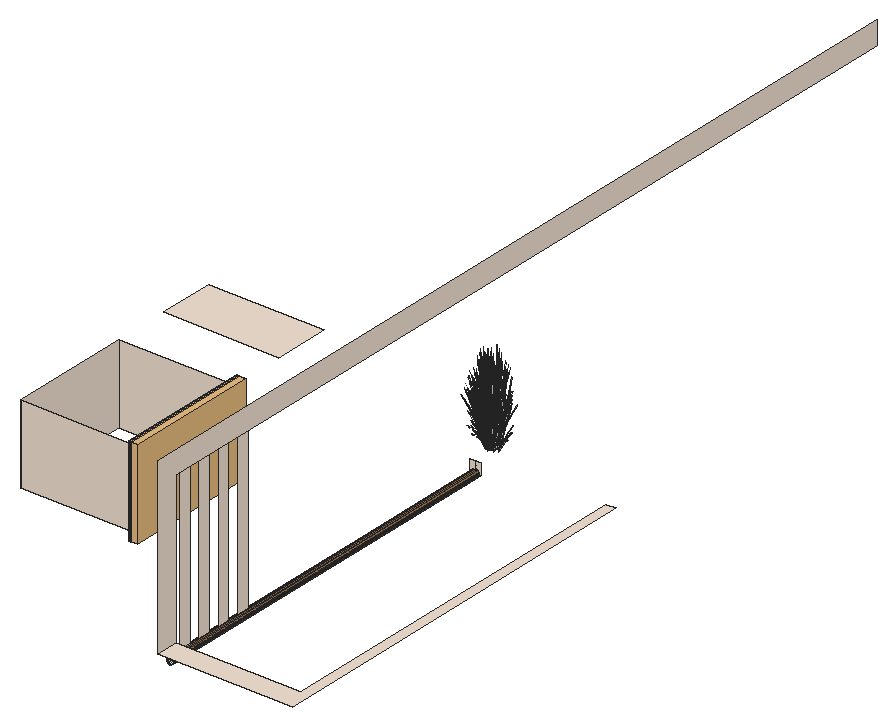
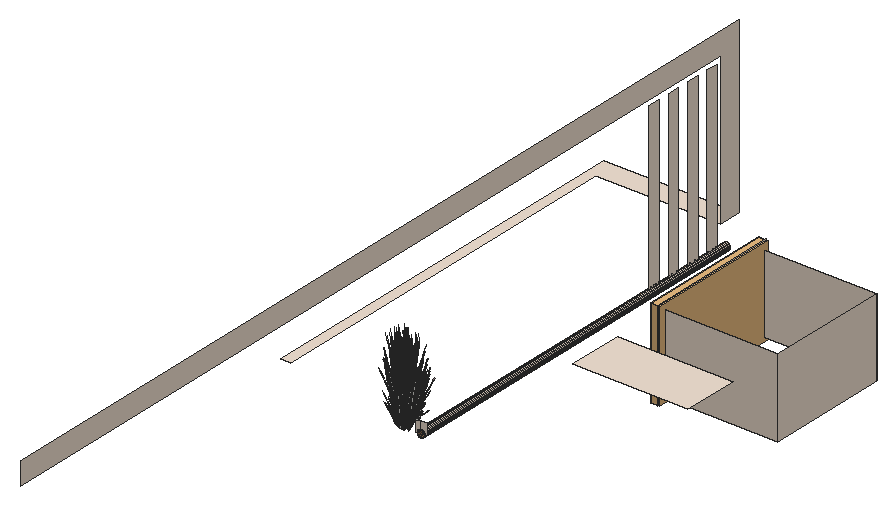
# SketchUp Ruby script. Lengths in inches.
U = 1.inch
M = Sketchup.active_model
def pt(a) = Geom::Point3d.new(a.map { |v| v * U })
def face(e, loops, mat)
  f = e.add_face(loops[0].map { |a| pt(a) })
  loops[1..].each { |l| e.add_face(l.map { |a| pt(a) }).erase! }
  f.material = f.back_material = mat if mat
  f
end
# faces: each face lists its corners as indices into pts; further lists are holes
def faces(e, pts, list, mat = nil) = list.each { |f| face(e, (f[0].is_a?(Array) ? f : [f]).map { |l| l.map { |i| pts[i] } }, mat) }
# xy, xz, yz: faces in a plane at the given z, y or x. An outline is a flat list of corners, or four numbers for a rectangle; further outlines are holes
def ring(l) = l.size == 4 ? [[l[0], l[1]], [l[2], l[1]], [l[2], l[3]], [l[0], l[3]]] : l.each_slice(2).to_a
def flat(e, list, mat, &to3) = list.each { |f| face(e, (f[0].is_a?(Array) ? f : [f]).map { |l| ring(l).map { |u, v| to3.(u, v) } }, mat) }
def xy(e, z, list, mat = nil) = flat(e, list, mat) { |x, y| [x, y, z] }
def xz(e, y, list, mat = nil) = flat(e, list, mat) { |x, z| [x, y, z] }
def yz(e, x, list, mat = nil) = flat(e, list, mat) { |y, z| [x, y, z] }
def lines(e, pts, list) = list.each { |a, b| e.add_line(pt(pts[a]), pt(pts[b])) }
# prism: a flat outline (further loops are holes) pulled along v
def prism(e, loops, v, mat = nil)
  f = face(e, loops, mat); d = Geom::Vector3d.new(v.map { |x| x * U })
  f.pushpull(f.normal.samedirection?(d) ? d.length : -d.length)
end
def box(e, o, s, mat = nil) = prism(e, [[o, [o[0] + s[0], o[1], o[2]], [o[0] + s[0], o[1] + s[1], o[2]], [o[0], o[1] + s[1], o[2]]]], [0, 0, s[2]], mat)
def at(x, y, z, deg = 0) = Geom::Transformation.translation(pt([x, y, z])) * Geom::Transformation.rotation(ORIGIN, Z_AXIS, deg.degrees)
def axes(o, x, y, z) = Geom::Transformation.new([*x, 0, *y, 0, *z, 0, *pt(o).to_a, 1])
def part(name) = M.definitions.add(name)
# library, detail: a bought-in or finely detailed component or shape, given as its bounding box
def library(name, o, s) = part(name).tap { |d| box(d.entities, o, s) }
def detail(e, o, s) = box(e.add_group.entities, o, s)
def put(e, d, t, mat = nil) = e.add_instance(d, t).tap { |i| i.material = mat if mat }
def group(e, t, mat = nil) = e.add_group.tap { |g| g.transformation = t; g.material = mat if mat }.entities
root = M.entities
M.materials.add("C01_Vanilla_Cream").color = [244, 228, 212]
M.materials.add("LightPink_Translucent").color = [144, 107, 117]
M.materials["LightPink_Translucent"].alpha = 0.75
M.materials.add("Wood_Floor_01_1K").color = [146, 111, 76]
c1 = library("Double casement window",[0,0,0],[5.02,56.42,60])
c2 = part("blade")
p = [[2.15,0.21,22],[0,0.17,0],[0.09,0.45,0],[2.18,0.31,22],[2.29,0.31,22],[0.38,0.45,0],
  [2.48,0.24,33],[2.49,0.24,33],[2.48,0.22,33]]
faces(c2.entities,p,[[0,1,2,3],[4,5,2,3],[6,3,4,7],[8,0,3,6]])
c3 = part("seeds")
p = [[0.3,-0.1,1.38],[-0.01,-0.03,1.59],[-0.01,-0.03,0.03],[0.14,-0.07,-0.07],[0.29,-0.03,3],[0.15,0.01,3.11]]
faces(c3.entities,p,[[0,1,2,3],[1,0,4,5]],"LightPink_Translucent")
c4 = part("blade with seeds")
put(c4.entities,c2,at(0,0,0))
put(c4.entities,c3,axes([2.4,0.25,30.99],[1.5799,-0.05474,1.17369],[-0.12525,1.92788,0.29478],[-0.07173,-0.02425,1.56792]))
xy(root,51.56,[[360,0,432,0,432,216,426.72,216,426.72,12,360,12]],"C01_Vanilla_Cream")
xy(root,93,[[226.53,171,288,201]],"C01_Vanilla_Cream")
xz(root,75,[[226.53,51,288,93]],"C01_Vanilla_Cream")
xz(root,141,[[226.53,51,288,93]],"C01_Vanilla_Cream")
xz(root,216,[[354,42,355,42,355.07,42.52,355.27,43,355.59,43.41,356,43.73,356.48,43.93,357,44,357,48,354,48],[359,42,360,42,360,48,357,48,357,44,357.52,43.93,358,43.73,358.41,43.41,358.73,43,358.93,42.52]],"C01_Vanilla_Cream")
yz(root,226.53,[[75,51,141,93]],"C01_Vanilla_Cream")
yz(root,288,[[[72,48,144,96],[109.5,51,141,93],[75,51,106.5,93]]],"C01_Vanilla_Cream")
yz(root,357,[[18.46,40,24.91,44],[31.37,40,37.83,44],[44.28,40,50.74,44],[57.2,40,63.65,44],[18.46,44,24.91,132],
  [31.37,44,37.83,132],[44.28,44,50.74,132],[57.2,44,63.65,132]],"C01_Vanilla_Cream")
yz(root,360,[[0,51.56,12,51.56,12,132,480,132,480,144,0,144]],"C01_Vanilla_Cream")
p = [[356.48,216,40.07],[357,216,40],[357,63.65,40],[357,57.2,40],[357,50.74,40],[357,44.28,40],
  [357,37.83,40],[357,31.37,40],[357,24.91,40],[357,18.46,40],[357,12,40],[356.48,12,40.07],
  [357.52,216,40.07],[357.52,12,40.07],[356,216,40.27],[356,12,40.27],[358,216,40.27],[358,12,40.27],
  [355.59,216,40.59],[355.59,12,40.59],[358.41,216,40.59],[358.41,12,40.59],[355.27,216,41],[355.27,12,41],
  [358.73,216,41],[358.73,12,41],[355.07,216,41.48],[355.07,12,41.48],[358.93,216,41.48],[358.93,12,41.48],
  [355,216,42],[355,12,42],[359,216,42],[359,12,42],[355.07,216,42.52],[355.07,12,42.52],
  [358.93,216,42.52],[358.93,12,42.52],[355.27,216,43],[355.27,12,43],[358.73,216,43],[358.73,12,43],
  [355.59,216,43.41],[355.59,12,43.41],[358.41,216,43.41],[358.41,12,43.41],[356,216,43.73],[356,12,43.73],
  [358,216,43.73],[358,12,43.73],[356.48,216,43.93],[356.48,12,43.93],[357.52,216,43.93],[357.52,12,43.93],
  [357,216,44],[357,12,44],[357,18.46,44],[357,24.91,44],[357,31.37,44],[357,37.83,44],
  [357,44.28,44],[357,50.74,44],[357,57.2,44],[357,63.65,44]]
faces(root,p,[[0,1,2,3,4,5,6,7,8,9,10,11],[14,0,11,15],[18,14,15,19],[22,18,19,23],[26,22,23,27],[30,26,27,31],[34,30,31,35],[38,34,35,39],
  [42,38,39,43],[46,42,43,47],[50,46,47,51],[54,50,51,55,56,57,58,59,60,61,62,63]],"C01_Vanilla_Cream")
faces(root,p,[[1,12,13,10,9,8,7,6,5,4,3,2],[12,16,17,13],[16,20,21,17],[20,24,25,21],[24,28,29,25],[28,32,33,29],[32,36,37,33],[36,40,41,37],
  [40,44,45,41],[44,48,49,45],[48,52,53,49],[52,54,63,62,61,60,59,58,57,56,55,53]],"Wood_Floor_01_1K")
put(root,c1,axes([286.7,72.24,48.3],[1,0,0],[0,1.27666,0],[0,0,0.79394]))
put(root,c4,axes([356.25,225,50.91],[0.12726,0.15818,1.28532],[-0.58807,0.13317,0.10393],[-0.13291,-0.24832,0.54946]))
put(root,c4,axes([357.22,223.95,51.54],[-0.08515,-0.06907,1.31208],[-0.56828,0.04379,-0.2075],[-0.0907,-0.16522,0.10523]))
put(root,c4,axes([358.54,224.77,49.94],[-0.15825,0.09972,1.07251],[-0.47395,-0.17454,-0.23066],[0.08785,-0.21706,0.45856]))
put(root,c4,axes([357.82,225.12,51.74],[-0.26572,-0.40059,-0.53284],[0.54698,-0.22325,0.0643],[-0.06214,-0.19355,0.75375]))
put(root,c4,axes([356.09,224.58,49.94],[-0.03371,0.16116,1.07251],[-0.49286,0.13491,-0.23066],[-0.11521,-0.20831,0.45856]))
put(root,c4,axes([357.36,224.23,49.12],[-0.09338,0.01775,1.32257],[-0.51641,-0.1998,-0.20205],[0.00867,-0.16666,0.22528]))
put(root,c4,axes([358.92,225.51,51.74],[0.01449,-0.45571,-0.53284],[0.61002,0.03061,0.0643],[0.06438,-0.19306,0.75375]))
put(root,c4,axes([359.77,224.8,51.54],[-0.00537,-0.09805,1.31208],[-0.45391,-0.28338,-0.2075],[0.07018,-0.17178,0.10523]))
put(root,c4,axes([357.87,224.78,51.39],[0.16784,-0.37886,-0.2656],[0.48968,0.1105,0.3429],[-0.0449,-0.15254,0.65611]))
put(root,c4,axes([358.24,225.28,50.91],[-0.10366,0.16934,1.28532],[-0.43488,-0.35044,0.10393],[0.19618,-0.21841,0.54946]))
put(root,c4,axes([359.65,224.44,51.53],[-0.05654,0.03763,1.33037],[-0.55396,-0.12696,-0.12571],[-0.02005,-0.16422,0.23543]))
put(root,c4,axes([357.62,225.04,51.51],[-0.54728,-0.1235,-0.38324],[0.18759,-0.42344,-0.29685],[-0.05018,-0.17048,0.7333]))
put(root,c4,axes([357.95,223.98,50.07],[0.07142,0.28728,0.86145],[-0.3962,-0.15911,0.63294],[0.04263,-0.1471,0.18974]))
put(root,c4,axes([358.8,225.36,51.51],[-0.39855,-0.33102,-0.38324],[0.42102,-0.2899,-0.29685],[0.06064,-0.16819,0.7333]))
put(root,c4,axes([356.64,223.72,51.53],[-0.01039,0.05905,1.33037],[-0.51226,0.21431,-0.12571],[-0.15074,-0.10955,0.23543]))
put(root,c4,axes([356.52,224.77,51.82],[0.62019,-0.12663,0.40322],[0.10763,0.49673,0.33247],[-0.14586,-0.1464,0.83437]))
put(root,c4,axes([357.93,224.86,51.55],[0.54859,0.1288,0.36002],[-0.18759,0.42344,0.29685],[-0.03297,-0.16652,0.74497]))
put(root,c4,axes([358.08,225.02,51.78],[-0.54481,0.22937,-0.0912],[-0.26773,-0.4071,-0.50621],[-0.07188,-0.17155,0.76918]))
put(root,c4,axes([359.22,225.53,51.78],[-0.61188,-0.02441,-0.0912],[0.01672,-0.46217,-0.50621],[0.0425,-0.178,0.76918]))
put(root,c4,axes([359.17,225.23,51.39],[0.3767,-0.25939,-0.2656],[0.3566,0.29618,0.3429],[0.05426,-0.15048,0.65611]))
put(root,c4,axes([355.92,224.32,50.07],[0.29042,0.17147,0.86145],[-0.42295,0.10307,0.63294],[-0.0905,-0.13178,0.18974]))
put(root,c4,axes([358.07,224.83,51.55],[0.41024,-0.16744,0.04823],[0.2008,0.30532,0.37966],[-0.03962,-0.13459,0.57892]))
put(root,c4,axes([356.62,225.23,51.74],[-0.47473,-0.23813,-0.53284],[0.33738,-0.41728,0.0643],[-0.172,-0.14218,0.75375]))
put(root,c4,axes([356.45,224.91,51.39],[-0.08599,-0.39682,-0.2656],[0.49155,-0.10478,0.3429],[-0.13203,-0.11372,0.65611]))
put(root,c4,axes([356.67,224.88,51.55],[0.25304,-0.31296,0.04823],[0.36033,0.18221,0.37966],[-0.11649,-0.10034,0.57892]))
put(root,c4,axes([355.6875,224.84,49.12],[-0.05393,0.0649,1.32257],[-0.545,0.13993,-0.20205],[-0.13166,-0.12729,0.22528]))
put(root,c4,axes([356.59,226.62,49.57],[-0.22864,-0.5052,-0.52377],[0.65862,-0.18195,-0.13747],[-0.02527,-0.17107,1.15612]))
put(root,c4,axes([355.4,225.49,50.91],[0.2068,0.08488,1.28532],[-0.42797,0.35609,0.10393],[-0.26673,-0.16064,0.54946]))
put(root,c4,axes([359.64,225.08,49.12],[-0.08333,-0.03881,1.32257],[-0.21404,-0.4336,-0.20205],[0.14439,-0.11767,0.22528]))
put(root,c4,axes([357.92,225.17,51.79],[-0.16784,0.37886,0.2656],[-0.48968,-0.1105,-0.3429],[-0.0449,-0.15254,0.65611]))
put(root,c4,axes([356.4,225.24,51.51],[-0.54938,0.11711,-0.38324],[-0.0961,-0.44351,-0.29685],[-0.14756,-0.1271,0.7333]))
put(root,c4,axes([359.17,225.33,51.55],[0.39645,0.33614,0.36002],[-0.42102,0.2899,0.29685],[0.07313,-0.15771,0.74497]))
put(root,c4,axes([356.78,224.85,52.07],[-0.37157,0.4723,-0.10215],[-0.5381,-0.2721,-0.56695],[-0.18705,-0.13344,0.86148]))
put(root,c4,axes([359.32,225.37,51.55],[0.45752,0.02296,0.04823],[-0.01254,0.34663,0.37966],[0.04787,-0.13278,0.57892]))
put(root,c4,axes([358.98,225.6,51.79],[-0.3767,0.25939,0.2656],[-0.3566,-0.29618,-0.3429],[0.05426,-0.15048,0.65611]))
put(root,c4,axes([359.64,226.3,51.74],[0.29081,-0.38873,-0.53284],[0.5096,0.27626,0.0643],[0.17364,-0.14084,0.75375]))
put(root,c4,axes([356.5,225.17,49.78],[-0.34808,-0.49367,0],[0.58235,-0.27531,-0.38706],[0.13264,-0.0627,1.22783]))
put(root,c4,axes([359.625,226.12,51.51],[-0.14302,-0.44985,-0.38324],[0.54163,-0.07869,-0.29685],[0.15522,-0.12083,0.7333]))
put(root,c4,axes([357.26,224.57,49.6],[-0.38473,0.28263,-0.02919],[-0.35252,-0.30954,-0.13237],[-0.02482,-0.08771,0.43661]))
put(root,c4,axes([355.36,224.71,51.54],[-0.11979,-0.00348,1.31208],[-0.38137,0.34775,-0.2075],[-0.20349,-0.07106,0.10523]))
put(root,c4,axes([359.88,226.44,51.78],[-0.515,-0.27165,-0.0912],[0.2967,-0.3934,-0.50621],[0.1455,-0.13675,0.76918]))
put(root,c4,axes([357.75,227.92,50.49],[0.48111,0.19866,1.13446],[-0.47133,0.42798,0.44862],[-0.21112,-0.25366,0.95105]))
put(root,c4,axes([356.75,225.24,51.79],[0.08599,0.39682,0.2656],[-0.49155,0.10478,-0.3429],[-0.13203,-0.11372,0.65611]))
put(root,c4,axes([355.24,226.55,49.51],[0,-0.49266,-0.37238],[0.62289,0,0],[0,-0.11221,1.18128]))
put(root,c4,axes([356.97,225.09,49.51],[0.52105,-0.24633,-0.37238],[0.31144,0.44171,0],[0.11867,-0.0561,1.18128]))
put(root,c4,axes([360.0625,225.94,49.94],[-0.19889,-0.01459,1.07251],[-0.20376,-0.39145,-0.23066],[0.24434,-0.11074,0.45856]))
put(root,c4,axes([355.27,225.5,51.82],[0.45978,-0.36358,0.40322],[0.39653,0.38611,0.33247],[-0.21571,-0.06707,0.83437]))
put(root,c4,axes([361.15,226.32,51.53],[-0.07272,-0.00374,1.33037],[-0.30197,-0.40092,-0.12571],[0.12127,-0.13182,0.23543]))
put(root,c4,axes([357.59,226.1,49.54],[0.375,-0.3703,-0.46765],[0.46584,0.33578,-0.12274],[0.15027,-0.09237,1.03225]))
put(root,c4,axes([360.29,225.22,50.07],[-0.18544,0.25079,0.86145],[-0.15939,-0.33694,0.63294],[0.15316,-0.08443,0.18974]))
put(root,c4,axes([360.03,226.17,51.39],[0.48462,-0.07041,-0.2656],[0.12797,0.4025,0.3429],[0.13888,-0.10811,0.65611]))
put(root,c4,axes([355.48,225.49,51.55],[0.02803,-0.37463,0.04823],[0.42332,0.01027,0.37966],[-0.16216,-0.0392,0.57892]))
put(root,c4,axes([356.93,226.75,49.66],[0.27012,-0.44393,-0.33554],[0.56127,0.21365,0.16149],[0,-0.10233,1.07733]))
put(root,c4,axes([355.32,225.61,51.39],[-0.31678,-0.30846,-0.2656],[0.36171,-0.29199,0.3429],[-0.18378,-0.04443,0.65611]))
put(root,c4,axes([357.18,226.53,50],[-0.06488,-0.56215,-0.21822],[0.6757,-0.03399,-0.37502],[0.11898,-0.07488,1.19781]))
put(root,c4,axes([355.51,226.5625,49.52],[0.38863,-0.30738,-0.23233],[0.38863,0.30738,0.23233],[0,-0.09901,1.0423]))
put(root,c4,axes([355.35,225.09,49.6],[-0.1606,0.40228,-0.02919],[-0.4943,-0.12375,-0.13237],[-0.07505,-0.0658,0.43661]))
put(root,c4,axes([359.63,226.4,51.79],[-0.48462,0.07041,0.2656],[-0.12797,-0.4025,-0.3429],[0.13888,-0.10811,0.65611]))
put(root,c4,axes([356.87,227.12,50],[-0.62699,-0.23507,-0.21822],[0.3019,-0.49615,-0.37502],[-0.0197,-0.12182,1.19781]))
put(root,c4,axes([355.08,226.92,49.78],[-0.69617,0,0],[0,-0.55062,-0.38706],[0,-0.12541,1.22783]))
put(root,c4,axes([355.2,225.94,49.94],[0.1087,0.13716,1.07251],[-0.25048,0.37284,-0.23066],[-0.25719,-0.08912,0.45856]))
put(root,c4,axes([357.09,225.29,49.52],[0.51941,0.1219,-0.23233],[-0.13078,0.42928,0.23233],[0.10471,-0.0495,1.0423]))
put(root,c4,axes([355.65,225.82,51.74],[-0.55654,-0.01186,-0.53284],[0.03738,-0.49951,0.0643],[-0.23578,-0.05271,0.75375]))
put(root,c4,axes([360.07,226.34,51.55],[0.3822,0.20719,0.04823],[-0.22252,0.29505,0.37966],[0.12254,-0.09539,0.57892]))
put(root,c4,axes([359.96,226.25,51.55],[0.13808,0.45342,0.36002],[-0.54163,0.07869,0.29685],[0.15963,-0.10664,0.74497]))
put(root,c4,axes([361.42,226.8,51.54],[0.07726,-0.07504,1.31208],[-0.09888,-0.46032,-0.2075],[0.19384,-0.08728,0.10523]))
put(root,c4,axes([355.625,226.78,49.75],[-0.51786,0.4142,0.23067],[-0.51817,-0.40984,-0.27369],[-0.01808,-0.11762,1.23664]))
put(root,c4,axes([354.9,225,51.53],[0.04127,0.04917,1.33037],[-0.19898,0.44196,-0.12571],[-0.20151,0.0032,0.23543]))
put(root,c4,axes([357.27,226.97,49.82],[0.6273,0.23878,0.18048],[-0.3019,0.49615,0.37502],[0,-0.11437,1.20407]))
put(root,c4,axes([357.03,227.64,49.83],[0.14756,-0.58378,-0.17572],[0.69966,0.10176,0.38453],[-0.12225,-0.08062,1.1733]))
put(root,c4,axes([355.47,225.92,51.51],[-0.40426,0.32635,-0.38324],[-0.35404,-0.34474,-0.29685],[-0.2054,-0.04965,0.7333]))
put(root,c4,axes([355.77,225.77,51.79],[0.31678,0.30846,0.2656],[-0.36171,0.29199,-0.3429],[-0.18378,-0.04443,0.65611]))
put(root,c4,axes([354.56,226.35,50.07],[0.35544,-0.03525,0.86145],[-0.22547,0.31061,0.63294],[-0.17565,-0.04659,0.18974]))
put(root,c4,axes([357.07,226.64,50.04],[-0.60457,0.03041,0.33554],[-0.05467,-0.50484,-0.16149],[0.10823,-0.05117,1.07733]))
put(root,c4,axes([355.68,225.58,51.78],[-0.02981,0.50103,-0.0912],[-0.56442,-0.01369,-0.50621],[-0.21738,-0.0348,0.76918]))
put(root,c4,axes([355.51,227.01,49.86],[0,0.49266,0.37238],[-0.62289,0,0],[0,-0.11221,1.18128]))
put(root,c4,axes([359.9,227.5,51.78],[-0.28012,-0.44611,-0.0912],[0.49717,-0.21923,-0.50621],[0.20951,-0.05886,0.76918]))
put(root,c4,axes([359.88,227.12,51.51],[0.15083,-0.44814,-0.38324],[0.51712,0.15361,-0.29685],[0.2082,-0.04109,0.7333]))
put(root,c4,axes([359.0625,225.29,49.78],[0.34808,-0.49367,0],[0.58235,0.27531,-0.38706],[0.13264,0.0627,1.22783]))
put(root,c4,axes([354.96,226.27,50.91],[0.23093,-0.01116,1.28532],[-0.15319,0.4836,0.10393],[-0.32909,-0.02991,0.54946]))
put(root,c4,axes([356.98,227.4,49.66],[-0.33445,-0.41351,-0.33554],[0.50659,-0.29119,0.16149],[-0.10823,-0.05117,1.07733]))
put(root,c4,axes([357.05,226.82,49.77],[0.24206,0.5509,0.34316],[-0.69162,0.19157,0.13466],[0.00845,-0.10123,1.19142]))
put(root,c4,axes([360.43,227.24,49.49],[-0.35858,0.05912,1.06187],[-0.05708,-0.47061,0.06078],[0.25115,-0.07123,0.60425]))
put(root,c4,axes([361.08,226.83,49.7],[-0.34516,-0.31503,-0.04866],[0.37803,-0.28865,-0.22062],[0.10711,-0.02032,0.72768]))
put(root,c4,axes([356.92,227.25,50.04],[-0.27012,0.44393,0.33554],[-0.56127,-0.21365,-0.16149],[0,-0.10233,1.07733]))
put(root,c4,axes([357.92,226.87,49.65],[0,-0.57005,0],[0.69617,0,0],[0,0,1.34592]))
put(root,c4,axes([358.76,225.55,49.86],[-0.52105,-0.24633,0.37238],[0.31144,-0.44171,0],[0.11867,0.0561,1.18128]))
put(root,c4,axes([359.78,227.28,51.74],[0.48922,-0.21758,-0.53284],[0.27264,0.44789,0.0643],[0.23638,-0.05088,0.75375]))
put(root,c4,axes([356.68,227.5625,49.54],[-0.57914,-0.08077,-0.46765],[0.12221,-0.49823,-0.12274],[-0.17283,-0.06037,1.03225]))
put(root,c4,axes([357.59,226.51,49.77],[-0.46162,0.4471,0.34316],[-0.54842,-0.39467,0.13466],[0.11129,-0.04462,1.19142]))
put(root,c4,axes([358.09,227.31,49.72],[-0.51786,-0.42404,-0.04598],[0.51817,-0.4243,0],[-0.01808,-0.01481,1.31678]))
put(root,c4,axes([356.79,225.77,49.86],[-0.16083,0.48962,0.13232],[-0.58854,-0.13856,0.26315],[0.10167,-0.00238,1.20305]))
put(root,c4,axes([359.71,227.37,51.79],[-0.46269,-0.13744,0.2656],[0.13495,-0.40096,-0.3429],[0.18628,-0.03677,0.65611]))
put(root,c4,axes([354.86,226.63,51.55],[0.15729,-0.44921,0.36002],[0.51712,0.15361,0.29685],[-0.20336,0.027,0.74497]))
put(root,c4,axes([356.54,226.17,49.2],[-0.548,0.19724,0.96696],[-0.17442,-0.56594,0.37572],[0.3365,0.00941,1.09981]))
put(root,c4,axes([358.01,226.32,49.96],[0.1074,-0.43968,0.1086],[0.52474,0.07632,-0.3101],[0.0955,0.04515,0.95058]))
put(root,c4,axes([354.83,226.51,51.55],[-0.20448,-0.33592,0.04823],[0.37288,-0.16442,0.37966],[-0.16437,0.03244,0.57892]))
put(root,c4,axes([357.11,227.36,49.77],[0.70367,0.1038,0.34316],[-0.1432,0.58624,0.13466],[-0.10283,-0.05661,1.19142]))
put(root,c4,axes([360.82,226.9375,49.12],[-0.0291,-0.0748,1.32257],[0.20181,-0.43752,-0.20205],[0.20357,-0.00629,0.22528]))
put(root,c4,axes([354.81,226.86,49.12],[0.01412,0.07764,1.32257],[-0.28464,0.40547,-0.20205],[-0.20218,-0.02044,0.22528]))
put(root,c4,axes([357.79,226.43,50.04],[-0.33445,-0.41351,0.33554],[0.50659,-0.29119,-0.16149],[0.10823,0.05117,1.07733]))
put(root,c4,axes([356.0625,228.32,49.52],[-0.13078,-0.42928,-0.23233],[0.51941,-0.1219,0.23233],[-0.10471,-0.0495,1.0423]))
put(root,c4,axes([356.73,228.3,49.86],[0.59825,-0.13076,0.13232],[0.14773,0.48663,0.26315],[-0.05336,-0.0709,1.20305]))
put(root,c4,axes([357.96,226.46,50],[0.56211,-0.32708,-0.21822],[0.3738,0.46216,-0.37502],[0.13869,0.04694,1.19781]))
put(root,c4,axes([360.2,227.32,51.39],[0.46269,0.13744,-0.2656],[-0.13495,0.40096,0.3429],[0.18628,-0.03677,0.65611]))
put(root,c4,axes([355.92,228.51,49.51],[-0.52105,-0.24633,-0.37238],[0.31144,-0.44171,0],[-0.11867,-0.0561,1.18128]))
put(root,c4,axes([359.38,225.59,49.51],[0.52105,0.24633,-0.37238],[-0.31144,0.44171,0],[0.11867,0.0561,1.18128]))
put(root,c4,axes([354.76,226.68,51.39],[-0.46269,-0.13744,-0.2656],[0.13495,-0.40096,0.3429],[-0.18628,0.03677,0.65611]))
put(root,c4,axes([358.39,227,49.65],[0.62289,0,0],[0,0.51004,0],[0,0,1.33805]))
put(root,c4,axes([357.33,227.64,50],[-0.56211,0.32708,-0.21822],[-0.3738,-0.46216,-0.37502],[-0.13869,-0.04694,1.19781]))
put(root,c4,axes([358.57,225.8,49.86],[-0.59825,0.13076,0.13232],[-0.14773,-0.48663,0.26315],[0.05336,0.0709,1.20305]))
put(root,c4,axes([358.93,226.83,50.91],[-0.23093,0.01116,1.28532],[0.15319,-0.4836,0.10393],[0.32909,0.02991,0.54946]))
put(root,c4,axes([359.23,225.77,49.52],[0.13078,0.42928,-0.23233],[-0.51941,0.1219,0.23233],[0.10471,0.0495,1.0423]))
put(root,c4,axes([360.13,227.49,51.55],[0.20448,0.33592,0.04823],[-0.37288,0.16442,0.37966],[0.16437,-0.03244,0.57892]))
put(root,c4,axes([358.1875,226.74,49.79],[-0.70367,-0.1038,0.36899],[0.1432,-0.58624,0.1448],[0.10283,0.05661,1.2811]))
put(root,c4,axes([360.09,227.37,51.55],[-0.15729,0.44921,0.36002],[-0.51712,-0.15361,0.29685],[0.20336,-0.027,0.74497]))
put(root,c4,axes([357.625,228.18,49.65],[-0.18165,-0.42474,0],[0.51872,-0.14874,0],[0,0,1.15778]))
put(root,c4,axes([357.28,227.78,49.96],[-0.1074,0.43968,0.1086],[-0.52474,-0.07632,-0.3101],[-0.0955,-0.04515,0.95058]))
put(root,c4,axes([355.24,226.64,51.79],[0.46269,0.13744,0.2656],[-0.13495,0.40096,-0.3429],[-0.18628,0.03677,0.65611]))
put(root,c4,axes([358.31,228.125,49.64],[0.5845,-0.16716,-0.14398],[0.20539,0.48152,0.00006],[0.06452,-0.01848,1.30423]))
put(root,c4,axes([358.51,228.32,49.86],[0.16083,-0.48962,0.13232],[0.58854,0.13856,0.26315],[-0.10167,0.00238,1.20305]))
put(root,c4,axes([358.375,227.21,49.66],[0.38863,0.31822,0],[-0.38863,0.31822,0],[0,0,1.2695]))
put(root,c4,axes([356.17,226.62,50.51],[0.15825,-0.07127,1.32798],[0.05457,0.4976,0.10393],[-0.34278,0.06603,0.47463]))
put(root,c4,axes([359.43,227.07,49.86],[-0.43742,-0.35886,0.13232],[0.44081,-0.34807,0.26315],[-0.04831,0.07329,1.20305]))
put(root,c4,axes([358.62,226.53,49.54],[0.57914,0.08077,-0.46765],[-0.12221,0.49823,-0.12274],[0.17283,0.06037,1.03225]))
put(root,c4,axes([361.18,227.4,50.07],[-0.34399,0.08133,0.86145],[0.16192,-0.33614,0.63294],[0.18249,0.023,0.18974]))
put(root,c4,axes([357.5,228.375,49.65],[-0.56127,-0.22118,0],[0.27012,-0.45959,0],[0,0,1.2203]))
put(root,c4,axes([357.96,227.79,49.85],[-0.54364,-0.39653,-0.18894],[0.45745,-0.44527,0.41347],[-0.14639,0.04639,1.26162]))
put(root,c4,axes([356.53,228.55,49.86],[0.52105,0.24633,0.37238],[-0.31144,0.44171,0],[-0.11867,-0.0561,1.18128]))
put(root,c4,axes([358.37,226.84,50.04],[0.27012,-0.44393,0.33554],[0.56127,0.21365,-0.16149],[0,0.10233,1.07733]))
put(root,c4,axes([361.02,228.83,51.53],[-0.05034,-0.04313,1.33037],[0.11012,-0.46232,-0.12571],[0.1983,-0.02954,0.23543]))
put(root,c4,axes([354.47,226.95,51.54],[-0.09091,0.06396,1.31208],[0.00773,0.46734,-0.2075],[-0.20839,0.06078,0.10523]))
put(root,c4,axes([358.27,227.1,49.72],[0,0.56976,-0.04228],[-0.69617,0,0],[0,0.01791,1.34526]))
put(root,c4,axes([355.07,226.89,51.51],[-0.15083,0.44814,-0.38324],[-0.51712,-0.15361,-0.29685],[-0.2082,0.04109,0.7333]))
put(root,c4,axes([355.05,226.5,51.78],[0.28012,0.44611,-0.0912],[-0.49717,0.21923,-0.50621],[-0.20951,0.05886,0.76918]))
put(root,c4,axes([358.32,226.69,49.66],[0.33445,0.41351,-0.33554],[-0.50659,0.29119,0.16149],[0.10823,0.05117,1.07733]))
put(root,c4,axes([360.58,228.44,50.95],[-0.10656,-0.41414,-0.02619],[0.50364,-0.09521,-0.11874],[0.10517,0.02626,0.39164]))
put(root,c4,axes([356.23,228.8,49.78],[-0.34808,0.49367,0],[-0.58235,-0.27531,-0.38706],[-0.13264,-0.0627,1.22783]))
put(root,c4,axes([359.27,228.43,51.78],[0.02981,-0.50103,-0.0912],[0.56442,0.01369,-0.50621],[0.21738,0.0348,0.76918]))
put(root,c4,axes([359.79,227.09,49.86],[0,-0.49266,0.37238],[0.62289,0,0],[0,0.11221,1.18128]))
put(root,c4,axes([358.23,227.46,50.04],[0.60457,-0.03041,0.33554],[0.05467,0.50484,-0.16149],[-0.10823,0.05117,1.07733]))
put(root,c4,axes([358.6,226.94,49.96],[0.51872,-0.14368,0.1086],[0.18165,0.41027,-0.3101],[0,0.09029,0.95058]))
put(root,c4,axes([359.1875,228.23,51.79],[-0.31678,-0.30846,0.2656],[0.36171,-0.29199,-0.3429],[0.18378,0.04443,0.65611]))
put(root,c4,axes([357.6875,227.7,49.66],[-0.60457,0.03041,-0.33554],[-0.05467,-0.50484,0.16149],[-0.10823,0.05117,1.07733]))
